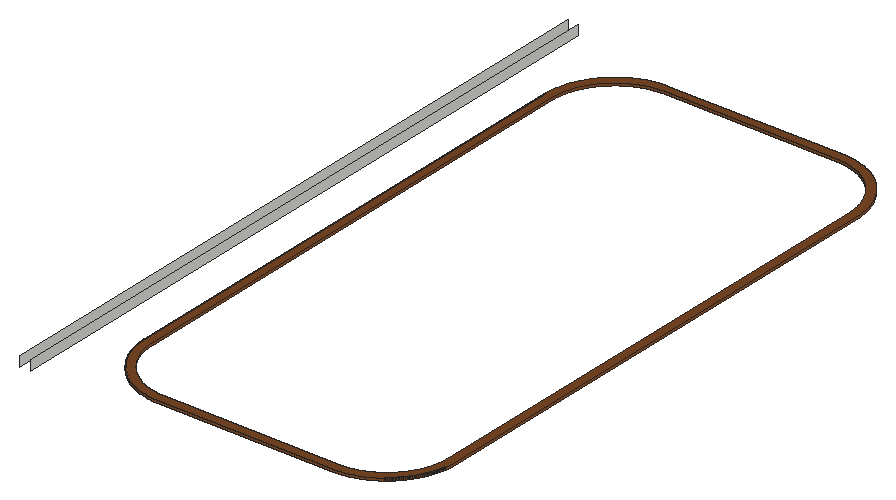
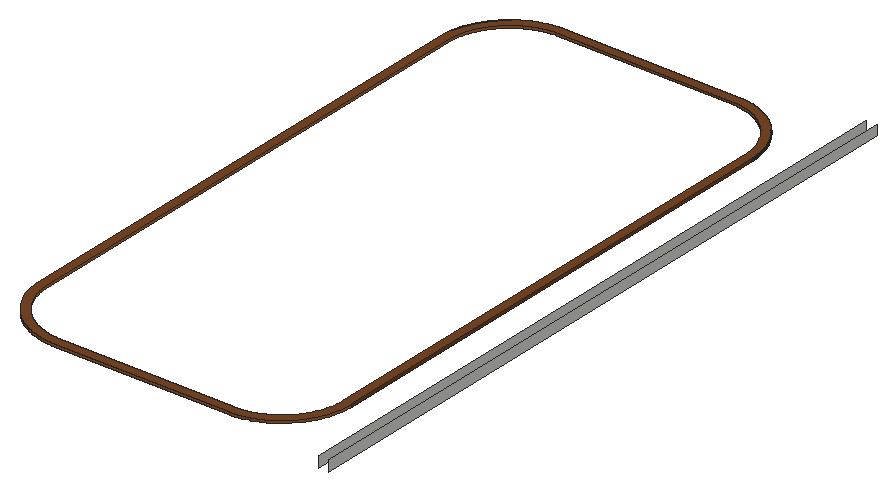
# SketchUp Ruby script. Lengths in inches.
U = 1.inch
M = Sketchup.active_model
def pt(a) = Geom::Point3d.new(a.map { |v| v * U })
def face(e, loops, mat)
  f = e.add_face(loops[0].map { |a| pt(a) })
  loops[1..].each { |l| e.add_face(l.map { |a| pt(a) }).erase! }
  f.material = f.back_material = mat if mat
  f
end
# faces: each face lists its corners as indices into pts; further lists are holes
def faces(e, pts, list, mat = nil) = list.each { |f| face(e, (f[0].is_a?(Array) ? f : [f]).map { |l| l.map { |i| pts[i] } }, mat) }
# xy, xz, yz: faces in a plane at the given z, y or x. An outline is a flat list of corners, or four numbers for a rectangle; further outlines are holes
def ring(l) = l.size == 4 ? [[l[0], l[1]], [l[2], l[1]], [l[2], l[3]], [l[0], l[3]]] : l.each_slice(2).to_a
def flat(e, list, mat, &to3) = list.each { |f| face(e, (f[0].is_a?(Array) ? f : [f]).map { |l| ring(l).map { |u, v| to3.(u, v) } }, mat) }
def xy(e, z, list, mat = nil) = flat(e, list, mat) { |x, y| [x, y, z] }
def xz(e, y, list, mat = nil) = flat(e, list, mat) { |x, z| [x, y, z] }
def yz(e, x, list, mat = nil) = flat(e, list, mat) { |y, z| [x, y, z] }
def lines(e, pts, list) = list.each { |a, b| e.add_line(pt(pts[a]), pt(pts[b])) }
# prism: a flat outline (further loops are holes) pulled along v
def prism(e, loops, v, mat = nil)
  f = face(e, loops, mat); d = Geom::Vector3d.new(v.map { |x| x * U })
  f.pushpull(f.normal.samedirection?(d) ? d.length : -d.length)
end
def box(e, o, s, mat = nil) = prism(e, [[o, [o[0] + s[0], o[1], o[2]], [o[0] + s[0], o[1] + s[1], o[2]], [o[0], o[1] + s[1], o[2]]]], [0, 0, s[2]], mat)
def at(x, y, z, deg = 0) = Geom::Transformation.translation(pt([x, y, z])) * Geom::Transformation.rotation(ORIGIN, Z_AXIS, deg.degrees)
def axes(o, x, y, z) = Geom::Transformation.new([*x, 0, *y, 0, *z, 0, *pt(o).to_a, 1])
def part(name) = M.definitions.add(name)
# library, detail: a bought-in or finely detailed component or shape, given as its bounding box
def library(name, o, s) = part(name).tap { |d| box(d.entities, o, s) }
def detail(e, o, s) = box(e.add_group.entities, o, s)
def put(e, d, t, mat = nil) = e.add_instance(d, t).tap { |i| i.material = mat if mat }
def group(e, t, mat = nil) = e.add_group.tap { |g| g.transformation = t; g.material = mat if mat }.entities
root = M.entities
M.materials.add("[Wood Veneer 01]3").color = [120, 70, 37]
xy(root,121,[[[92.65,43.5,92.29,43.52,92.12,43.53,91.94,43.54,91.76,43.56,91.59,43.57,91.41,43.59,91.24,43.62,91.0625,43.64,90.89,43.67,90.71,43.69,90.54,43.73,90.37,43.76,90.19,43.79,89.85,43.87,89.68,43.92,89.51,43.96,88.83,44.16,88.66,44.22,88.49,44.27,88.33,44.33,88.16,44.4,88,44.46,87.83,44.53,87.35,44.74,87.1875,44.82,87.03,44.89,86.71,45.05,86.56,45.14,86.4,45.22,85.8,45.58,85.5,45.78,85.35,45.875,85.21,45.98,85.06,46.08,84.92,46.18,84.5,46.51,84.37,46.62,84.23,46.73,83.45,47.45,82.73,48.23,82.62,48.37,82.51,48.5,82.18,48.92,82.08,49.06,81.98,49.21,81.875,49.35,81.78,49.5,81.58,49.8,81.22,50.4,81.14,50.56,81.05,50.71,80.89,51.03,80.82,51.1875,80.74,51.35,80.53,51.83,80.46,52,80.4,52.16,80.33,52.33,80.27,52.49,80.22,52.66,80.16,52.83,79.96,53.51,79.92,53.68,79.87,53.85,79.79,54.19,79.76,54.37,79.73,54.54,79.69,54.71,79.67,54.89,79.64,55.0625,79.62,55.24,79.59,55.41,79.57,55.59,79.56,55.76,79.54,55.94,79.53,56.12,79.52,56.29,79.5,56.65,79.5,153.35,79.52,153.71,79.53,153.88,79.54,154.06,79.56,154.24,79.57,154.41,79.59,154.59,79.62,154.76,79.64,154.9375,79.67,155.11,79.69,155.29,79.73,155.46,79.76,155.63,79.79,155.81,79.87,156.15,79.92,156.32,79.96,156.49,80.16,157.17,80.22,157.34,80.27,157.51,80.33,157.67,80.4,157.84,80.46,158,80.53,158.17,80.74,158.65,80.82,158.8125,80.89,158.97,81.05,159.29,81.14,159.44,81.22,159.6,81.58,160.2,81.78,160.5,81.875,160.65,81.98,160.79,82.08,160.94,82.18,161.08,82.51,161.5,82.62,161.63,82.73,161.77,83.45,162.55,84.23,163.27,84.37,163.38,84.5,163.49,84.92,163.82,85.06,163.92,85.21,164.02,85.35,164.125,85.5,164.22,85.8,164.42,86.4,164.78,86.56,164.86,86.71,164.95,87.03,165.11,87.1875,165.18,87.35,165.26,87.83,165.47,88,165.54,88.16,165.6,88.33,165.67,88.49,165.73,88.66,165.78,88.83,165.84,89.51,166.04,89.68,166.08,89.85,166.13,90.19,166.21,90.37,166.24,90.54,166.27,90.71,166.31,90.89,166.33,91.0625,166.36,91.24,166.38,91.41,166.41,91.59,166.43,91.76,166.44,91.94,166.46,92.12,166.47,92.29,166.48,92.65,166.5,126.35,166.5,126.71,166.48,126.88,166.47,127.06,166.46,127.24,166.44,127.41,166.43,127.59,166.41,127.76,166.38,127.9375,166.36,128.11,166.33,128.29,166.31,128.46,166.27,128.63,166.24,128.81,166.21,129.15,166.13,129.32,166.08,129.49,166.04,130.17,165.84,130.34,165.78,130.51,165.73,130.67,165.67,130.84,165.6,131,165.54,131.17,165.47,131.65,165.26,131.8125,165.18,131.97,165.11,132.29,164.95,132.44,164.86,132.6,164.78,133.2,164.42,133.5,164.22,133.65,164.125,133.79,164.02,133.94,163.92,134.08,163.82,134.5,163.49,134.63,163.38,134.77,163.27,135.55,162.55,136.27,161.77,136.38,161.63,136.49,161.5,136.82,161.08,136.92,160.94,137.02,160.79,137.125,160.65,137.22,160.5,137.42,160.2,137.78,159.6,137.86,159.44,137.95,159.29,138.11,158.97,138.18,158.8125,138.26,158.65,138.47,158.17,138.54,158,138.6,157.84,138.67,157.67,138.73,157.51,138.78,157.34,138.84,157.17,139.04,156.49,139.08,156.32,139.13,156.15,139.21,155.81,139.24,155.63,139.27,155.46,139.31,155.29,139.33,155.11,139.36,154.9375,139.38,154.76,139.41,154.59,139.43,154.41,139.44,154.24,139.46,154.06,139.47,153.88,139.48,153.71,139.5,153.35,139.5,56.65,139.48,56.29,139.47,56.12,139.46,55.94,139.44,55.76,139.43,55.59,139.41,55.41,139.38,55.24,139.36,55.0625,139.33,54.89,139.31,54.71,139.27,54.54,139.24,54.37,139.21,54.19,139.13,53.85,139.08,53.68,139.04,53.51,138.84,52.83,138.78,52.66,138.73,52.49,138.67,52.33,138.6,52.16,138.54,52,138.47,51.83,138.26,51.35,138.18,51.1875,138.11,51.03,137.95,50.71,137.86,50.56,137.78,50.4,137.42,49.8,137.22,49.5,137.125,49.35,137.02,49.21,136.92,49.06,136.82,48.92,136.49,48.5,136.38,48.37,136.27,48.23,135.55,47.45,134.77,46.73,134.63,46.62,134.5,46.51,134.08,46.18,133.94,46.08,133.79,45.98,133.65,45.875,133.5,45.78,133.2,45.58,132.6,45.22,132.44,45.14,132.29,45.05,131.97,44.89,131.8125,44.82,131.65,44.74,131.17,44.53,131,44.46,130.84,44.4,130.67,44.33,130.51,44.27,130.34,44.22,130.17,44.16,129.49,43.96,129.32,43.92,129.15,43.87,128.81,43.79,128.63,43.76,128.46,43.73,128.29,43.69,128.11,43.67,127.9375,43.64,127.76,43.62,127.59,43.59,127.41,43.57,127.24,43.56,127.06,43.54,126.88,43.53,126.71,43.52,126.35,43.5],[92.6875,45,126.3125,45,126.47,45.01,126.63,45.02,126.78,45.03,127.1,45.05,127.25,45.07,127.41,45.08,127.57,45.1,127.72,45.125,127.88,45.15,128.03,45.17,128.1875,45.2,128.34,45.23,128.49,45.26,128.65,45.3,128.8,45.33,128.95,45.37,129.11,45.41,129.41,45.49,129.86,45.64,130.01,45.6875,130.15,45.74,130.3,45.8,130.45,45.85,130.59,45.91,130.74,45.97,130.88,46.04,131.02,46.1,131.17,46.17,131.73,46.45,131.86,46.53,132,46.61,132.14,46.6875,132.27,46.77,132.4,46.85,132.54,46.9375,132.67,47.02,132.93,47.2,133.05,47.29,133.18,47.38,133.31,47.48,133.43,47.58,133.55,47.67,133.67,47.77,133.91,47.98,134.03,48.08,134.15,48.1875,134.26,48.3,134.375,48.4,134.49,48.51,134.6,48.625,134.7,48.74,134.8125,48.85,134.92,48.97,135.02,49.09,135.23,49.33,135.33,49.45,135.42,49.57,135.52,49.69,135.62,49.82,135.71,49.95,135.8,50.07,135.98,50.33,136.0625,50.46,136.15,50.6,136.23,50.73,136.3125,50.86,136.39,51,136.47,51.14,136.55,51.27,136.83,51.83,136.9,51.98,136.96,52.12,137.03,52.26,137.09,52.41,137.15,52.55,137.2,52.7,137.26,52.85,137.3125,52.99,137.36,53.14,137.51,53.59,137.59,53.89,137.63,54.05,137.67,54.2,137.7,54.35,137.74,54.51,137.77,54.66,137.8,54.8125,137.83,54.97,137.85,55.12,137.875,55.28,137.9,55.43,137.92,55.59,137.93,55.75,137.95,55.9,137.97,56.22,137.98,56.37,137.99,56.53,138,56.6875,138,153.3125,137.99,153.47,137.98,153.63,137.97,153.78,137.95,154.1,137.93,154.25,137.92,154.41,137.9,154.57,137.875,154.72,137.85,154.88,137.83,155.03,137.8,155.1875,137.77,155.34,137.74,155.49,137.7,155.65,137.67,155.8,137.63,155.95,137.59,156.11,137.51,156.41,137.36,156.86,137.3125,157.01,137.26,157.15,137.2,157.3,137.15,157.45,137.09,157.59,137.03,157.74,136.96,157.88,136.9,158.02,136.83,158.17,136.55,158.73,136.47,158.86,136.39,159,136.3125,159.14,136.23,159.27,136.15,159.4,136.0625,159.54,135.98,159.67,135.8,159.93,135.71,160.05,135.62,160.18,135.52,160.31,135.42,160.43,135.33,160.55,135.23,160.67,135.02,160.91,134.92,161.03,134.8125,161.15,134.7,161.26,134.6,161.375,134.49,161.49,134.375,161.6,134.26,161.7,134.15,161.8125,134.03,161.92,133.91,162.02,133.67,162.23,133.55,162.33,133.43,162.42,133.31,162.52,133.18,162.62,133.05,162.71,132.93,162.8,132.67,162.98,132.54,163.0625,132.4,163.15,132.27,163.23,132.14,163.3125,132,163.39,131.86,163.47,131.73,163.55,131.17,163.83,131.02,163.9,130.88,163.96,130.74,164.03,130.59,164.09,130.45,164.15,130.3,164.2,130.15,164.26,130.01,164.3125,129.86,164.36,129.41,164.51,129.11,164.59,128.95,164.63,128.8,164.67,128.65,164.7,128.49,164.74,128.34,164.77,128.1875,164.8,128.03,164.83,127.88,164.85,127.72,164.875,127.57,164.9,127.41,164.92,127.25,164.93,127.1,164.95,126.78,164.97,126.63,164.98,126.47,164.99,126.3125,165,92.6875,165,92.53,164.99,92.37,164.98,92.22,164.97,91.9,164.95,91.75,164.93,91.59,164.92,91.43,164.9,91.28,164.875,91.12,164.85,90.97,164.83,90.8125,164.8,90.66,164.77,90.51,164.74,90.35,164.7,90.2,164.67,90.05,164.63,89.89,164.59,89.59,164.51,89.14,164.36,88.99,164.3125,88.85,164.26,88.7,164.2,88.55,164.15,88.41,164.09,88.26,164.03,88.12,163.96,87.98,163.9,87.83,163.83,87.27,163.55,87.14,163.47,87,163.39,86.86,163.3125,86.73,163.23,86.6,163.15,86.46,163.0625,86.33,162.98,86.07,162.8,85.95,162.71,85.82,162.62,85.69,162.52,85.57,162.42,85.45,162.33,85.33,162.23,85.09,162.02,84.97,161.92,84.85,161.8125,84.74,161.7,84.625,161.6,84.51,161.49,84.4,161.375,84.3,161.26,84.1875,161.15,84.08,161.03,83.98,160.91,83.77,160.67,83.67,160.55,83.58,160.43,83.48,160.31,83.38,160.18,83.29,160.05,83.2,159.93,83.02,159.67,82.9375,159.54,82.85,159.4,82.77,159.27,82.6875,159.14,82.61,159,82.53,158.86,82.45,158.73,82.17,158.17,82.1,158.02,82.04,157.88,81.97,157.74,81.91,157.59,81.85,157.45,81.8,157.3,81.74,157.15,81.6875,157.01,81.64,156.86,81.49,156.41,81.41,156.11,81.37,155.95,81.33,155.8,81.3,155.65,81.26,155.49,81.23,155.34,81.2,155.1875,81.17,155.03,81.15,154.88,81.125,154.72,81.1,154.57,81.08,154.41,81.07,154.25,81.05,154.1,81.03,153.78,81.02,153.63,81.01,153.47,81,153.3125,81,56.6875,81.01,56.53,81.02,56.37,81.03,56.22,81.05,55.9,81.07,55.75,81.08,55.59,81.1,55.43,81.125,55.28,81.15,55.12,81.17,54.97,81.2,54.8125,81.23,54.66,81.26,54.51,81.3,54.35,81.33,54.2,81.37,54.05,81.41,53.89,81.49,53.59,81.64,53.14,81.6875,52.99,81.74,52.85,81.8,52.7,81.85,52.55,81.91,52.41,81.97,52.26,82.04,52.12,82.1,51.98,82.17,51.83,82.45,51.27,82.53,51.14,82.61,51,82.6875,50.86,82.77,50.73,82.85,50.6,82.9375,50.46,83.02,50.33,83.2,50.07,83.29,49.95,83.38,49.82,83.48,49.69,83.58,49.57,83.67,49.45,83.77,49.33,83.98,49.09,84.08,48.97,84.1875,48.85,84.3,48.74,84.4,48.625,84.51,48.51,84.625,48.4,84.74,48.3,84.85,48.1875,84.97,48.08,85.09,47.98,85.33,47.77,85.45,47.67,85.57,47.58,85.69,47.48,85.82,47.38,85.95,47.29,86.07,47.2,86.33,47.02,86.46,46.9375,86.6,46.85,86.73,46.77,86.86,46.6875,87,46.61,87.14,46.53,87.27,46.45,87.83,46.17,87.98,46.1,88.12,46.04,88.26,45.97,88.41,45.91,88.55,45.85,88.7,45.8,88.85,45.74,88.99,45.6875,89.14,45.64,89.59,45.49,89.89,45.41,90.05,45.37,90.2,45.33,90.35,45.3,90.51,45.26,90.66,45.23,90.8125,45.2,90.97,45.17,91.12,45.15,91.28,45.125,91.43,45.1,91.59,45.08,91.75,45.07,91.9,45.05,92.22,45.03,92.37,45.02,92.53,45.01]]],"[Wood Veneer 01]3")
xy(root,121.5,[[[92.65,43.5,126.35,43.5,126.71,43.52,126.88,43.53,127.06,43.54,127.24,43.56,127.41,43.57,127.59,43.59,127.76,43.62,127.9375,43.64,128.11,43.67,128.29,43.69,128.46,43.73,128.63,43.76,128.81,43.79,129.15,43.87,129.32,43.92,129.49,43.96,130.17,44.16,130.34,44.22,130.51,44.27,130.67,44.33,130.84,44.4,131,44.46,131.17,44.53,131.65,44.74,131.8125,44.82,131.97,44.89,132.29,45.05,132.44,45.14,132.6,45.22,133.2,45.58,133.5,45.78,133.65,45.875,133.79,45.98,133.94,46.08,134.08,46.18,134.5,46.51,134.63,46.62,134.77,46.73,135.55,47.45,136.27,48.23,136.38,48.37,136.49,48.5,136.82,48.92,136.92,49.06,137.02,49.21,137.125,49.35,137.22,49.5,137.42,49.8,137.78,50.4,137.86,50.56,137.95,50.71,138.11,51.03,138.18,51.1875,138.26,51.35,138.47,51.83,138.54,52,138.6,52.16,138.67,52.33,138.73,52.49,138.78,52.66,138.84,52.83,139.04,53.51,139.08,53.68,139.13,53.85,139.21,54.19,139.24,54.37,139.27,54.54,139.31,54.71,139.33,54.89,139.36,55.0625,139.38,55.24,139.41,55.41,139.43,55.59,139.44,55.76,139.46,55.94,139.47,56.12,139.48,56.29,139.5,56.65,139.5,153.35,139.48,153.71,139.47,153.88,139.46,154.06,139.44,154.24,139.43,154.41,139.41,154.59,139.38,154.76,139.36,154.9375,139.33,155.11,139.31,155.29,139.27,155.46,139.24,155.63,139.21,155.81,139.13,156.15,139.08,156.32,139.04,156.49,138.84,157.17,138.78,157.34,138.73,157.51,138.67,157.67,138.6,157.84,138.54,158,138.47,158.17,138.26,158.65,138.18,158.8125,138.11,158.97,137.95,159.29,137.86,159.44,137.78,159.6,137.42,160.2,137.22,160.5,137.125,160.65,137.02,160.79,136.92,160.94,136.82,161.08,136.49,161.5,136.38,161.63,136.27,161.77,135.55,162.55,134.77,163.27,134.63,163.38,134.5,163.49,134.08,163.82,133.94,163.92,133.79,164.02,133.65,164.125,133.5,164.22,133.2,164.42,132.6,164.78,132.44,164.86,132.29,164.95,131.97,165.11,131.8125,165.18,131.65,165.26,131.17,165.47,131,165.54,130.84,165.6,130.67,165.67,130.51,165.73,130.34,165.78,130.17,165.84,129.49,166.04,129.32,166.08,129.15,166.13,128.81,166.21,128.63,166.24,128.46,166.27,128.29,166.31,128.11,166.33,127.9375,166.36,127.76,166.38,127.59,166.41,127.41,166.43,127.24,166.44,127.06,166.46,126.88,166.47,126.71,166.48,126.35,166.5,92.65,166.5,92.29,166.48,92.12,166.47,91.94,166.46,91.76,166.44,91.59,166.43,91.41,166.41,91.24,166.38,91.0625,166.36,90.89,166.33,90.71,166.31,90.54,166.27,90.37,166.24,90.19,166.21,89.85,166.13,89.68,166.08,89.51,166.04,88.83,165.84,88.66,165.78,88.49,165.73,88.33,165.67,88.16,165.6,88,165.54,87.83,165.47,87.35,165.26,87.1875,165.18,87.03,165.11,86.71,164.95,86.56,164.86,86.4,164.78,85.8,164.42,85.5,164.22,85.35,164.125,85.21,164.02,85.06,163.92,84.92,163.82,84.5,163.49,84.37,163.38,84.23,163.27,83.45,162.55,82.73,161.77,82.62,161.63,82.51,161.5,82.18,161.08,82.08,160.94,81.98,160.79,81.875,160.65,81.78,160.5,81.58,160.2,81.22,159.6,81.14,159.44,81.05,159.29,80.89,158.97,80.82,158.8125,80.74,158.65,80.53,158.17,80.46,158,80.4,157.84,80.33,157.67,80.27,157.51,80.22,157.34,80.16,157.17,79.96,156.49,79.92,156.32,79.87,156.15,79.79,155.81,79.76,155.63,79.73,155.46,79.69,155.29,79.67,155.11,79.64,154.9375,79.62,154.76,79.59,154.59,79.57,154.41,79.56,154.24,79.54,154.06,79.53,153.88,79.52,153.71,79.5,153.35,79.5,56.65,79.52,56.29,79.53,56.12,79.54,55.94,79.56,55.76,79.57,55.59,79.59,55.41,79.62,55.24,79.64,55.0625,79.67,54.89,79.69,54.71,79.73,54.54,79.76,54.37,79.79,54.19,79.87,53.85,79.92,53.68,79.96,53.51,80.16,52.83,80.22,52.66,80.27,52.49,80.33,52.33,80.4,52.16,80.46,52,80.53,51.83,80.74,51.35,80.82,51.1875,80.89,51.03,81.05,50.71,81.14,50.56,81.22,50.4,81.58,49.8,81.78,49.5,81.875,49.35,81.98,49.21,82.08,49.06,82.18,48.92,82.51,48.5,82.62,48.37,82.73,48.23,83.45,47.45,84.23,46.73,84.37,46.62,84.5,46.51,84.92,46.18,85.06,46.08,85.21,45.98,85.35,45.875,85.5,45.78,85.8,45.58,86.4,45.22,86.56,45.14,86.71,45.05,87.03,44.89,87.1875,44.82,87.35,44.74,87.83,44.53,88,44.46,88.16,44.4,88.33,44.33,88.49,44.27,88.66,44.22,88.83,44.16,89.51,43.96,89.68,43.92,89.85,43.87,90.19,43.79,90.37,43.76,90.54,43.73,90.71,43.69,90.89,43.67,91.0625,43.64,91.24,43.62,91.41,43.59,91.59,43.57,91.76,43.56,91.94,43.54,92.12,43.53,92.29,43.52],[92.6875,45,92.53,45.01,92.37,45.02,92.22,45.03,91.9,45.05,91.75,45.07,91.59,45.08,91.43,45.1,91.28,45.125,91.12,45.15,90.97,45.17,90.8125,45.2,90.66,45.23,90.51,45.26,90.35,45.3,90.2,45.33,90.05,45.37,89.89,45.41,89.59,45.49,89.14,45.64,88.99,45.6875,88.85,45.74,88.7,45.8,88.55,45.85,88.41,45.91,88.26,45.97,88.12,46.04,87.98,46.1,87.83,46.17,87.27,46.45,87.14,46.53,87,46.61,86.86,46.6875,86.73,46.77,86.6,46.85,86.46,46.9375,86.33,47.02,86.07,47.2,85.95,47.29,85.82,47.38,85.69,47.48,85.57,47.58,85.45,47.67,85.33,47.77,85.09,47.98,84.97,48.08,84.85,48.1875,84.74,48.3,84.625,48.4,84.51,48.51,84.4,48.625,84.3,48.74,84.1875,48.85,84.08,48.97,83.98,49.09,83.77,49.33,83.67,49.45,83.58,49.57,83.48,49.69,83.38,49.82,83.29,49.95,83.2,50.07,83.02,50.33,82.9375,50.46,82.85,50.6,82.77,50.73,82.6875,50.86,82.61,51,82.53,51.14,82.45,51.27,82.17,51.83,82.1,51.98,82.04,52.12,81.97,52.26,81.91,52.41,81.85,52.55,81.8,52.7,81.74,52.85,81.6875,52.99,81.64,53.14,81.49,53.59,81.41,53.89,81.37,54.05,81.33,54.2,81.3,54.35,81.26,54.51,81.23,54.66,81.2,54.8125,81.17,54.97,81.15,55.12,81.125,55.28,81.1,55.43,81.08,55.59,81.07,55.75,81.05,55.9,81.03,56.22,81.02,56.37,81.01,56.53,81,56.6875,81,153.3125,81.01,153.47,81.02,153.63,81.03,153.78,81.05,154.1,81.07,154.25,81.08,154.41,81.1,154.57,81.125,154.72,81.15,154.88,81.17,155.03,81.2,155.1875,81.23,155.34,81.26,155.49,81.3,155.65,81.33,155.8,81.37,155.95,81.41,156.11,81.49,156.41,81.64,156.86,81.6875,157.01,81.74,157.15,81.8,157.3,81.85,157.45,81.91,157.59,81.97,157.74,82.04,157.88,82.1,158.02,82.17,158.17,82.45,158.73,82.53,158.86,82.61,159,82.6875,159.14,82.77,159.27,82.85,159.4,82.9375,159.54,83.02,159.67,83.2,159.93,83.29,160.05,83.38,160.18,83.48,160.31,83.58,160.43,83.67,160.55,83.77,160.67,83.98,160.91,84.08,161.03,84.1875,161.15,84.3,161.26,84.4,161.375,84.51,161.49,84.625,161.6,84.74,161.7,84.85,161.8125,84.97,161.92,85.09,162.02,85.33,162.23,85.45,162.33,85.57,162.42,85.69,162.52,85.82,162.62,85.95,162.71,86.07,162.8,86.33,162.98,86.46,163.0625,86.6,163.15,86.73,163.23,86.86,163.3125,87,163.39,87.14,163.47,87.27,163.55,87.83,163.83,87.98,163.9,88.12,163.96,88.26,164.03,88.41,164.09,88.55,164.15,88.7,164.2,88.85,164.26,88.99,164.3125,89.14,164.36,89.59,164.51,89.89,164.59,90.05,164.63,90.2,164.67,90.35,164.7,90.51,164.74,90.66,164.77,90.8125,164.8,90.97,164.83,91.12,164.85,91.28,164.875,91.43,164.9,91.59,164.92,91.75,164.93,91.9,164.95,92.22,164.97,92.37,164.98,92.53,164.99,92.6875,165,126.3125,165,126.47,164.99,126.63,164.98,126.78,164.97,127.1,164.95,127.25,164.93,127.41,164.92,127.57,164.9,127.72,164.875,127.88,164.85,128.03,164.83,128.1875,164.8,128.34,164.77,128.49,164.74,128.65,164.7,128.8,164.67,128.95,164.63,129.11,164.59,129.41,164.51,129.86,164.36,130.01,164.3125,130.15,164.26,130.3,164.2,130.45,164.15,130.59,164.09,130.74,164.03,130.88,163.96,131.02,163.9,131.17,163.83,131.73,163.55,131.86,163.47,132,163.39,132.14,163.3125,132.27,163.23,132.4,163.15,132.54,163.0625,132.67,162.98,132.93,162.8,133.05,162.71,133.18,162.62,133.31,162.52,133.43,162.42,133.55,162.33,133.67,162.23,133.91,162.02,134.03,161.92,134.15,161.8125,134.26,161.7,134.375,161.6,134.49,161.49,134.6,161.375,134.7,161.26,134.8125,161.15,134.92,161.03,135.02,160.91,135.23,160.67,135.33,160.55,135.42,160.43,135.52,160.31,135.62,160.18,135.71,160.05,135.8,159.93,135.98,159.67,136.0625,159.54,136.15,159.4,136.23,159.27,136.3125,159.14,136.39,159,136.47,158.86,136.55,158.73,136.83,158.17,136.9,158.02,136.96,157.88,137.03,157.74,137.09,157.59,137.15,157.45,137.2,157.3,137.26,157.15,137.3125,157.01,137.36,156.86,137.51,156.41,137.59,156.11,137.63,155.95,137.67,155.8,137.7,155.65,137.74,155.49,137.77,155.34,137.8,155.1875,137.83,155.03,137.85,154.88,137.875,154.72,137.9,154.57,137.92,154.41,137.93,154.25,137.95,154.1,137.97,153.78,137.98,153.63,137.99,153.47,138,153.3125,138,56.6875,137.99,56.53,137.98,56.37,137.97,56.22,137.95,55.9,137.93,55.75,137.92,55.59,137.9,55.43,137.875,55.28,137.85,55.12,137.83,54.97,137.8,54.8125,137.77,54.66,137.74,54.51,137.7,54.35,137.67,54.2,137.63,54.05,137.59,53.89,137.51,53.59,137.36,53.14,137.3125,52.99,137.26,52.85,137.2,52.7,137.15,52.55,137.09,52.41,137.03,52.26,136.96,52.12,136.9,51.98,136.83,51.83,136.55,51.27,136.47,51.14,136.39,51,136.3125,50.86,136.23,50.73,136.15,50.6,136.0625,50.46,135.98,50.33,135.8,50.07,135.71,49.95,135.62,49.82,135.52,49.69,135.42,49.57,135.33,49.45,135.23,49.33,135.02,49.09,134.92,48.97,134.8125,48.85,134.7,48.74,134.6,48.625,134.49,48.51,134.375,48.4,134.26,48.3,134.15,48.1875,134.03,48.08,133.91,47.98,133.67,47.77,133.55,47.67,133.43,47.58,133.31,47.48,133.18,47.38,133.05,47.29,132.93,47.2,132.67,47.02,132.54,46.9375,132.4,46.85,132.27,46.77,132.14,46.6875,132,46.61,131.86,46.53,131.73,46.45,131.17,46.17,131.02,46.1,130.88,46.04,130.74,45.97,130.59,45.91,130.45,45.85,130.3,45.8,130.15,45.74,130.01,45.6875,129.86,45.64,129.41,45.49,129.11,45.41,128.95,45.37,128.8,45.33,128.65,45.3,128.49,45.26,128.34,45.23,128.1875,45.2,128.03,45.17,127.88,45.15,127.72,45.125,127.57,45.1,127.41,45.08,127.25,45.07,127.1,45.05,126.78,45.03,126.63,45.02,126.47,45.01,126.3125,45]]],"[Wood Veneer 01]3")
yz(root,69.75,[[39.22,121,170.78,123]])
yz(root,71.75,[[39.29,121,170.71,123]])
yz(root,79.5,[[56.65,121,56.82,121.5],[56.82,121,57,121.5],[57,121,153,121.5]],"[Wood Veneer 01]3")
p = [[134.22,46.29,121],[134.36,46.4,121],[134.36,46.4,121.5],[134.22,46.29,121.5],[84.5,46.51,121],[84.64,46.4,121],
  [84.64,46.4,121.5],[84.5,46.51,121.5],[134.5,46.51,121],[134.5,46.51,121.5],[84.37,46.62,121],[84.37,46.62,121.5],
  [134.63,46.62,121],[134.63,46.62,121.5],[84.23,46.73,121],[84.23,46.73,121.5],[134.77,46.73,121],[134.77,46.73,121.5],
  [84.1,46.85,121],[84.1,46.85,121.5],[134.9,46.85,121],[134.9,46.85,121.5],[83.97,46.97,121],[83.97,46.97,121.5],
  [135.03,46.97,121],[135.03,46.97,121.5],[83.84,47.09,121],[83.84,47.09,121.5],[135.16,47.09,121],[135.16,47.09,121.5],
  [83.71,47.21,121],[83.71,47.21,121.5],[135.29,47.21,121],[135.29,47.21,121.5],[83.58,47.33,121],[83.58,47.33,121.5],
  [135.42,47.33,121],[135.42,47.33,121.5],[83.45,47.45,121],[83.45,47.45,121.5],[135.55,47.45,121],[135.55,47.45,121.5],
  [83.33,47.58,121],[83.33,47.58,121.5],[135.67,47.58,121],[135.67,47.58,121.5],[83.21,47.71,121],[83.21,47.71,121.5],
  [135.79,47.71,121],[135.79,47.71,121.5],[83.09,47.84,121],[83.09,47.84,121.5],[135.91,47.84,121],[135.91,47.84,121.5],
  [82.97,47.97,121],[82.97,47.97,121.5],[136.03,47.97,121],[136.03,47.97,121.5],[82.85,48.1,121],[82.85,48.1,121.5],
  [136.15,48.1,121],[136.15,48.1,121.5],[82.73,48.23,121],[82.73,48.23,121.5],[136.27,48.23,121],[136.27,48.23,121.5],
  [82.62,48.37,121],[82.62,48.37,121.5],[136.38,48.37,121],[136.38,48.37,121.5],[82.51,48.5,121],[82.51,48.5,121.5],
  [136.49,48.5,121],[136.49,48.5,121.5],[82.4,48.64,121],[82.4,48.64,121.5],[136.6,48.64,121],[136.6,48.64,121.5],
  [82.29,48.78,121],[82.29,48.78,121.5],[136.71,48.78,121],[136.71,48.78,121.5],[82.18,48.92,121],[82.18,48.92,121.5],
  [136.82,48.92,121],[136.82,48.92,121.5],[82.08,49.06,121],[82.08,49.06,121.5],[136.92,49.06,121],[136.92,49.06,121.5],
  [81.98,49.21,121],[81.98,49.21,121.5],[137.02,49.21,121],[137.02,49.21,121.5],[81.875,49.35,121],[81.875,49.35,121.5],
  [137.125,49.35,121],[137.125,49.35,121.5],[81.78,49.5,121],[81.78,49.5,121.5],[137.22,49.5,121],[137.22,49.5,121.5],
  [81.68,49.65,121],[81.68,49.65,121.5],[137.32,49.65,121],[137.32,49.65,121.5],[81.58,49.8,121],[81.58,49.8,121.5],
  [137.42,49.8,121],[137.42,49.8,121.5],[81.49,49.95,121],[81.49,49.95,121.5],[137.51,49.95,121],[137.51,49.95,121.5],
  [81.4,50.1,121],[81.4,50.1,121.5],[137.6,50.1,121],[137.6,50.1,121.5],[81.31,50.25,121],[81.31,50.25,121.5],
  [137.69,50.25,121],[137.69,50.25,121.5],[81.22,50.4,121],[81.22,50.4,121.5],[137.78,50.4,121],[137.78,50.4,121.5],
  [81.14,50.56,121],[81.14,50.56,121.5],[137.86,50.56,121],[137.86,50.56,121.5],[81.05,50.71,121],[81.05,50.71,121.5],
  [137.95,50.71,121],[137.95,50.71,121.5],[80.97,50.87,121],[80.97,50.87,121.5],[138.03,50.87,121],[138.03,50.87,121.5],
  [80.89,51.03,121],[80.89,51.03,121.5],[138.11,51.03,121],[138.11,51.03,121.5],[80.82,51.1875,121],[80.82,51.1875,121.5],
  [138.18,51.1875,121],[138.18,51.1875,121.5],[80.74,51.35,121],[80.74,51.35,121.5],[138.26,51.35,121],[138.26,51.35,121.5],
  [80.67,51.51,121],[80.67,51.51,121.5],[138.33,51.51,121],[138.33,51.51,121.5],[80.6,51.67,121],[80.6,51.67,121.5],
  [138.4,51.67,121],[138.4,51.67,121.5],[80.53,51.83,121],[80.53,51.83,121.5],[138.47,51.83,121],[138.47,51.83,121.5],
  [80.46,52,121],[80.46,52,121.5],[138.54,52,121],[138.54,52,121.5],[80.4,52.16,121],[80.4,52.16,121.5],
  [138.6,52.16,121],[138.6,52.16,121.5],[80.33,52.33,121],[80.33,52.33,121.5],[138.67,52.33,121],[138.67,52.33,121.5],
  [80.27,52.49,121],[80.27,52.49,121.5],[138.73,52.49,121],[138.73,52.49,121.5],[80.22,52.66,121],[80.22,52.66,121.5],
  [138.78,52.66,121],[138.78,52.66,121.5],[80.16,52.83,121],[80.16,52.83,121.5],[138.84,52.83,121],[138.84,52.83,121.5],
  [80.11,53,121],[80.11,53,121.5],[138.89,53,121],[138.89,53,121.5],[80.06,53.17,121],[80.06,53.17,121.5],
  [138.94,53.17,121],[138.94,53.17,121.5],[80.01,53.34,121],[80.01,53.34,121.5],[138.99,53.34,121],[138.99,53.34,121.5],
  [79.96,53.51,121],[79.96,53.51,121.5],[139.04,53.51,121],[139.04,53.51,121.5],[79.92,53.68,121],[79.92,53.68,121.5],
  [139.08,53.68,121],[139.08,53.68,121.5],[79.87,53.85,121],[79.87,53.85,121.5],[139.13,53.85,121],[139.13,53.85,121.5],
  [79.83,54.02,121],[79.83,54.02,121.5],[139.17,54.02,121],[139.17,54.02,121.5],[79.79,54.19,121],[79.79,54.19,121.5],
  [139.21,54.19,121],[139.21,54.19,121.5],[79.76,54.37,121],[79.76,54.37,121.5],[139.24,54.37,121],[139.24,54.37,121.5],
  [79.73,54.54,121],[79.73,54.54,121.5],[79.69,54.71,121],[79.69,54.71,121.5],[79.67,54.89,121],[79.67,54.89,121.5],
  [79.64,55.0625,121],[79.64,55.0625,121.5],[79.62,55.24,121],[79.62,55.24,121.5],[79.59,55.41,121],[79.59,55.41,121.5],
  [79.57,55.59,121],[79.57,55.59,121.5],[79.56,55.76,121],[79.56,55.76,121.5],[79.54,55.94,121],[79.54,55.94,121.5],
  [79.53,56.12,121],[79.53,56.12,121.5],[79.52,56.29,121],[79.52,56.29,121.5],[79.51,56.47,121],[79.51,56.47,121.5],
  [79.5,56.65,121],[79.5,56.65,121.5]]
faces(root,p,[[0,1,2,3],[4,5,6,7],[1,8,9,2],[10,4,7,11],[8,12,13,9],[14,10,11,15],[12,16,17,13],[18,14,15,19],
  [16,20,21,17],[22,18,19,23],[20,24,25,21],[26,22,23,27],[24,28,29,25],[30,26,27,31],[28,32,33,29],[34,30,31,35],
  [32,36,37,33],[38,34,35,39],[36,40,41,37],[42,38,39,43],[40,44,45,41],[46,42,43,47],[44,48,49,45],[50,46,47,51],
  [48,52,53,49],[54,50,51,55],[52,56,57,53],[58,54,55,59],[56,60,61,57],[62,58,59,63],[60,64,65,61],[66,62,63,67],
  [64,68,69,65],[70,66,67,71],[68,72,73,69],[74,70,71,75],[72,76,77,73],[78,74,75,79],[76,80,81,77],[82,78,79,83],
  [80,84,85,81],[86,82,83,87],[84,88,89,85],[90,86,87,91],[88,92,93,89],[94,90,91,95],[92,96,97,93],[98,94,95,99],
  [96,100,101,97],[102,98,99,103],[100,104,105,101],[106,102,103,107],[104,108,109,105],[110,106,107,111],[108,112,113,109],[114,110,111,115],
  [112,116,117,113],[118,114,115,119],[116,120,121,117],[122,118,119,123],[120,124,125,121],[126,122,123,127],[124,128,129,125],[130,126,127,131],
  [128,132,133,129],[134,130,131,135],[132,136,137,133],[138,134,135,139],[136,140,141,137],[142,138,139,143],[140,144,145,141],[146,142,143,147],
  [144,148,149,145],[150,146,147,151],[148,152,153,149],[154,150,151,155],[152,156,157,153],[158,154,155,159],[156,160,161,157],[162,158,159,163],
  [160,164,165,161],[166,162,163,167],[164,168,169,165],[170,166,167,171],[168,172,173,169],[174,170,171,175],[172,176,177,173],[178,174,175,179],
  [176,180,181,177],[182,178,179,183],[180,184,185,181],[186,182,183,187],[184,188,189,185],[190,186,187,191],[188,192,193,189],[194,190,191,195],
  [192,196,197,193],[198,194,195,199],[196,200,201,197],[202,198,199,203],[200,204,205,201],[206,202,203,207],[204,208,209,205],[210,206,207,211],
  [208,212,213,209],[214,210,211,215],[212,216,217,213],[218,214,215,219],[216,220,221,217],[222,218,219,223],[224,222,223,225],[226,224,225,227],
  [228,226,227,229],[230,228,229,231],[232,230,231,233],[234,232,233,235],[236,234,235,237],[238,236,237,239],[240,238,239,241],[242,240,241,243],
  [244,242,243,245],[246,244,245,247]],"[Wood Veneer 01]3")
